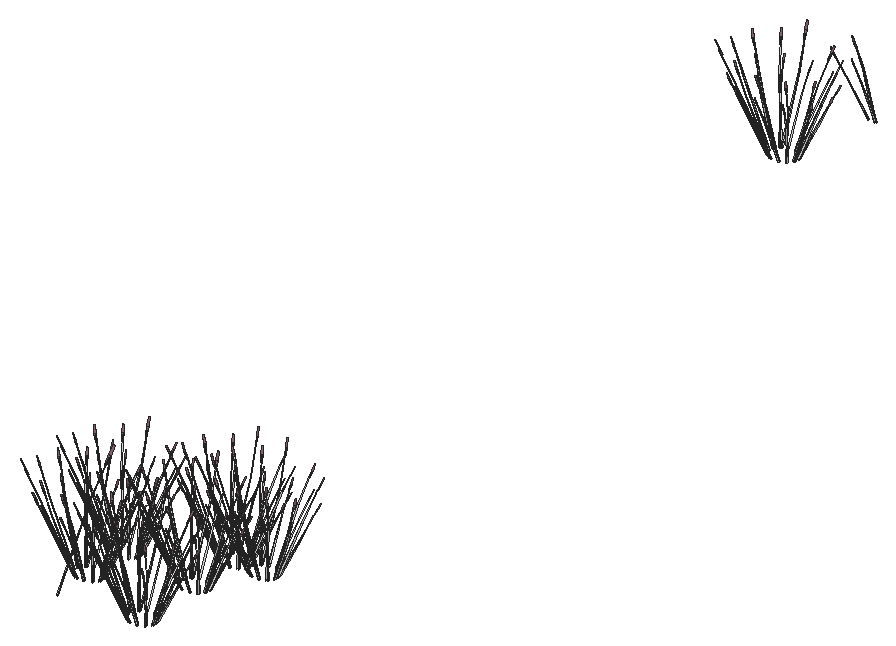
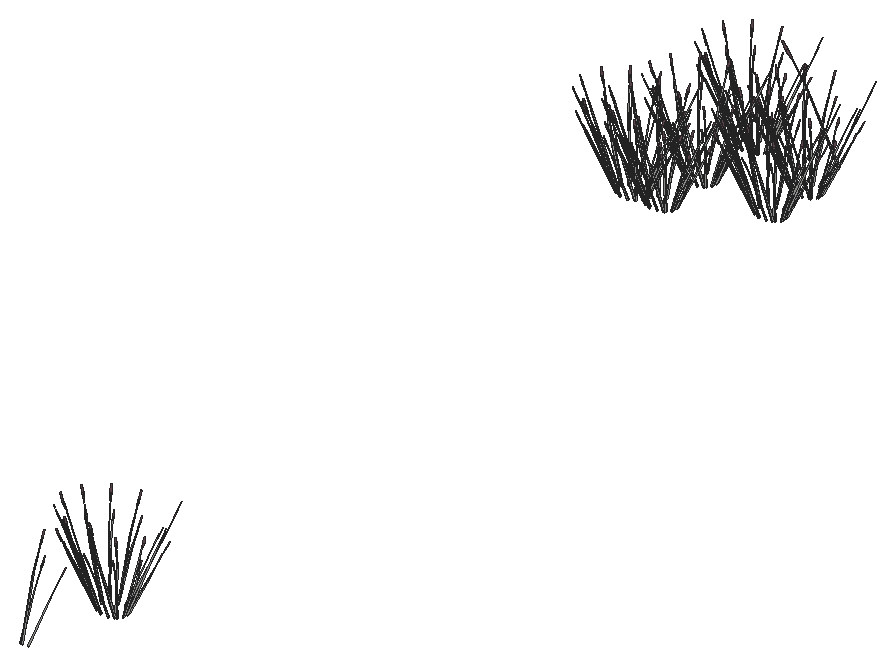
# SketchUp Ruby script. Lengths in inches.
U = 1.inch
M = Sketchup.active_model
def pt(a) = Geom::Point3d.new(a.map { |v| v * U })
def face(e, loops, mat)
  f = e.add_face(loops[0].map { |a| pt(a) })
  loops[1..].each { |l| e.add_face(l.map { |a| pt(a) }).erase! }
  f.material = f.back_material = mat if mat
  f
end
# faces: each face lists its corners as indices into pts; further lists are holes
def faces(e, pts, list, mat = nil) = list.each { |f| face(e, (f[0].is_a?(Array) ? f : [f]).map { |l| l.map { |i| pts[i] } }, mat) }
# xy, xz, yz: faces in a plane at the given z, y or x. An outline is a flat list of corners, or four numbers for a rectangle; further outlines are holes
def ring(l) = l.size == 4 ? [[l[0], l[1]], [l[2], l[1]], [l[2], l[3]], [l[0], l[3]]] : l.each_slice(2).to_a
def flat(e, list, mat, &to3) = list.each { |f| face(e, (f[0].is_a?(Array) ? f : [f]).map { |l| ring(l).map { |u, v| to3.(u, v) } }, mat) }
def xy(e, z, list, mat = nil) = flat(e, list, mat) { |x, y| [x, y, z] }
def xz(e, y, list, mat = nil) = flat(e, list, mat) { |x, z| [x, y, z] }
def yz(e, x, list, mat = nil) = flat(e, list, mat) { |y, z| [x, y, z] }
def lines(e, pts, list) = list.each { |a, b| e.add_line(pt(pts[a]), pt(pts[b])) }
# prism: a flat outline (further loops are holes) pulled along v
def prism(e, loops, v, mat = nil)
  f = face(e, loops, mat); d = Geom::Vector3d.new(v.map { |x| x * U })
  f.pushpull(f.normal.samedirection?(d) ? d.length : -d.length)
end
def box(e, o, s, mat = nil) = prism(e, [[o, [o[0] + s[0], o[1], o[2]], [o[0] + s[0], o[1] + s[1], o[2]], [o[0], o[1] + s[1], o[2]]]], [0, 0, s[2]], mat)
def at(x, y, z, deg = 0) = Geom::Transformation.translation(pt([x, y, z])) * Geom::Transformation.rotation(ORIGIN, Z_AXIS, deg.degrees)
def axes(o, x, y, z) = Geom::Transformation.new([*x, 0, *y, 0, *z, 0, *pt(o).to_a, 1])
def part(name) = M.definitions.add(name)
# library, detail: a bought-in or finely detailed component or shape, given as its bounding box
def library(name, o, s) = part(name).tap { |d| box(d.entities, o, s) }
def detail(e, o, s) = box(e.add_group.entities, o, s)
def put(e, d, t, mat = nil) = e.add_instance(d, t).tap { |i| i.material = mat if mat }
def group(e, t, mat = nil) = e.add_group.tap { |g| g.transformation = t; g.material = mat if mat }.entities
root = M.entities
M.materials.add("LightPink_Translucent").color = [144, 107, 117]
c1 = part("blade")
p = [[2.15,0.21,22],[0,0.17,0],[0.09,0.45,0],[2.18,0.31,22],[2.29,0.31,22],[0.38,0.45,0],
  [2.48,0.24,33],[2.49,0.24,33],[2.48,0.22,33]]
faces(c1.entities,p,[[0,1,2,3],[4,5,2,3],[6,3,4,7],[8,0,3,6]])
c2 = part("seeds")
p = [[0.3,-0.1,1.38],[-0.01,-0.03,1.59],[-0.01,-0.03,0.03],[0.14,-0.07,-0.07],[0.29,-0.03,3],[0.15,0.01,3.11]]
faces(c2.entities,p,[[0,1,2,3],[1,0,4,5]],"LightPink_Translucent")
c3 = part("blade with seeds")
put(c3.entities,c1,at(0,0,0))
put(c3.entities,c2,axes([2.4,0.25,30.99],[1.5799,-0.05474,1.17369],[-0.12525,1.92788,0.29478],[-0.07173,-0.02425,1.56792]))
put(root,c3,axes([64.49,21.74,46.73],[1.20755,0.27075,0.48003],[-0.41292,0.89013,0.3958],[-0.07257,-0.35005,0.9933]))
put(root,c3,axes([64.8125,21.67,46.73],[0.90301,-0.35198,0.0643],[0.44199,0.64184,0.50621],[-0.08721,-0.28293,0.77189]))
put(root,c3,axes([61.72,21.77,46.73],[0.55698,-0.6579,0.0643],[0.79316,0.38303,0.50621],[-0.25643,-0.21093,0.77189]))
put(root,c3,axes([67.23,22.73,46.73],[0.87265,0.70663,0.48003],[-0.92674,0.60943,0.3958],[0.16097,-0.33153,0.9933]))
put(root,c3,axes([61.97,21.7,47.43],[-0.81789,0.99285,-0.13619],[-1.18445,-0.572,-0.75594],[-0.41173,-0.28051,1.14864]))
put(root,c3,axes([67.55,22.8,46.73],[1.00708,0.04826,0.0643],[-0.02761,0.72867,0.50621],[0.10538,-0.27912,0.77189]))
put(root,c3,axes([59.1,23.0625,46.73],[0.06171,-0.78753,0.0643],[0.9318,0.02159,0.50621],[-0.35694,-0.08241,0.77189]))
put(root,c3,axes([69.21,24.84,46.73],[0.8413,0.43556,0.0643],[-0.48981,0.62025,0.50621],[0.26973,-0.20053,0.77189]))
put(root,c3,axes([68.97,24.66,46.73],[0.30393,0.95317,0.48003],[-1.19224,0.16542,0.3958],[0.35138,-0.22417,0.9933]))
put(root,c3,axes([57.75,25.46,46.73],[0.34623,-0.9443,0.48003],[1.13828,0.3229,0.3958],[-0.44763,0.05675,0.9933]))
put(root,c3,axes([57.66,25.21,46.73],[-0.4501,-0.70615,0.0643],[0.82077,-0.34564,0.50621],[-0.36181,0.0682,0.77189]))
put(root,c3,axes([69.33,27.26,46.73],[0.4501,0.70615,0.0643],[-0.82077,0.34564,0.50621],[0.36181,-0.0682,0.77189]))
put(root,c3,axes([69.25,27.01,46.73],[-0.34623,0.9443,0.48003],[-1.13828,-0.3229,0.3958],[0.44763,-0.05675,0.9933]))
put(root,c3,axes([33.02,33.74,46.73],[1.20755,0.27075,0.48003],[-0.41292,0.89013,0.3958],[-0.07257,-0.35005,0.9933]))
put(root,c3,axes([33.34,33.67,46.73],[0.90301,-0.35198,0.0643],[0.44199,0.64184,0.50621],[-0.08721,-0.28293,0.77189]))
put(root,c3,axes([30.25,33.77,46.73],[0.55698,-0.6579,0.0643],[0.79316,0.38303,0.50621],[-0.25643,-0.21093,0.77189]))
put(root,c3,axes([32.82,21.08,46.72],[-1.05895,-0.53811,1.38283],[1.11816,-0.83781,0.59665],[0.34166,0.5049,1.33663]))
put(root,c3,axes([35.76,34.73,46.73],[0.87265,0.70663,0.48003],[-0.92674,0.60943,0.3958],[0.16097,-0.33153,0.9933]))
put(root,c3,axes([30.5,33.7,47.43],[-0.81789,0.99285,-0.13619],[-1.18445,-0.572,-0.75594],[-0.41173,-0.28051,1.14864]))
put(root,c3,axes([36.08,34.8,46.73],[1.00708,0.04826,0.0643],[-0.02761,0.72867,0.50621],[0.10538,-0.27912,0.77189]))
put(root,c3,axes([58.02,27.81,46.73],[-0.30393,-0.95317,0.48003],[1.19224,-0.16542,0.3958],[-0.35138,0.22417,0.9933]))
put(root,c3,axes([57.79,27.63,46.73],[-0.8413,-0.43556,0.0643],[0.48981,-0.62025,0.50621],[-0.26973,0.20053,0.77189]))
put(root,c3,axes([67.9,29.4,46.73],[-0.06171,0.78753,0.0643],[-0.9318,-0.02159,0.50621],[0.35694,0.08241,0.77189]))
put(root,c3,axes([67.98,29.15,46.73],[-0.90362,0.68241,0.48003],[-0.77932,-0.72471,0.3958],[0.42395,0.12588,0.9933]))
put(root,c3,axes([27.63,35.0625,46.73],[0.06171,-0.78753,0.0643],[0.9318,0.02159,0.50621],[-0.35694,-0.08241,0.77189]))
put(root,c3,axes([37.74,36.84,46.73],[0.8413,0.43556,0.0643],[-0.48981,0.62025,0.50621],[0.26973,-0.20053,0.77189]))
put(root,c3,axes([37.5,36.66,46.73],[0.30393,0.95317,0.48003],[-1.19224,0.16542,0.3958],[0.35138,-0.22417,0.9933]))
put(root,c3,axes([59.44,29.67,46.73],[-1.00708,-0.04826,0.0643],[0.02761,-0.72867,0.50621],[-0.10538,0.27912,0.77189]))
put(root,c3,axes([59.77,29.74,46.73],[-0.87265,-0.70663,0.48003],[0.92674,-0.60943,0.3958],[-0.16097,0.33153,0.9933]))
put(root,c3,axes([65.28,30.7,46.73],[-0.55698,0.6579,0.0643],[-0.79316,-0.38303,0.50621],[0.25643,0.21093,0.77189]))
put(root,c3,axes([65.51,30.52,46.73],[-1.21888,0.23767,0.48003],[-0.21154,-0.93233,0.3958],[0.28666,0.27478,0.9933]))
put(root,c3,axes([62.1875,30.8,46.73],[-0.90301,0.35198,0.0643],[-0.44199,-0.64184,0.50621],[0.08721,0.28293,0.77189]))
put(root,c3,axes([59.67,29.33,47.4],[1.34686,0.05131,-0.13498],[-0.03681,0.97156,-0.74919],[-0.09356,0.37418,1.13838]))
put(root,c3,axes([26.28,37.46,46.73],[0.34623,-0.9443,0.48003],[1.13828,0.3229,0.3958],[-0.44763,0.05675,0.9933]))
put(root,c3,axes([26.19,37.21,46.73],[-0.4501,-0.70615,0.0643],[0.82077,-0.34564,0.50621],[-0.36181,0.0682,0.77189]))
put(root,c3,axes([37.86,39.26,46.73],[0.4501,0.70615,0.0643],[-0.82077,0.34564,0.50621],[0.36181,-0.0682,0.77189]))
put(root,c3,axes([37.78,39.01,46.73],[-0.34623,0.9443,0.48003],[-1.13828,-0.3229,0.3958],[0.44763,-0.05675,0.9933]))
put(root,c3,axes([26.55,39.81,46.73],[-0.30393,-0.95317,0.48003],[1.19224,-0.16542,0.3958],[-0.35138,0.22417,0.9933]))
put(root,c3,axes([26.32,39.63,46.73],[-0.8413,-0.43556,0.0643],[0.48981,-0.62025,0.50621],[-0.26973,0.20053,0.77189]))
put(root,c3,axes([64.28,49.02,46.73],[1.20755,0.27075,0.48003],[-0.41292,0.89013,0.3958],[-0.07257,-0.35005,0.9933]))
put(root,c3,axes([64.6,48.96,46.73],[0.90301,-0.35198,0.0643],[0.44199,0.64184,0.50621],[-0.08721,-0.28293,0.77189]))
put(root,c3,axes([36.42,41.4,46.73],[-0.06171,0.78753,0.0643],[-0.9318,-0.02159,0.50621],[0.35694,0.08241,0.77189]))
put(root,c3,axes([36.51,41.15,46.73],[-0.90362,0.68241,0.48003],[-0.77932,-0.72471,0.3958],[0.42395,0.12588,0.9933]))
put(root,c3,axes([61.51,49.06,46.73],[0.55698,-0.6579,0.0643],[0.79316,0.38303,0.50621],[-0.25643,-0.21093,0.77189]))
put(root,c3,axes([67.02,50.01,46.73],[0.87265,0.70663,0.48003],[-0.92674,0.60943,0.3958],[0.16097,-0.33153,0.9933]))
put(root,c3,axes([61.76,48.99,47.43],[-0.81789,0.99285,-0.13619],[-1.18445,-0.572,-0.75594],[-0.41173,-0.28051,1.14864]))
put(root,c3,axes([67.35,50.08,46.73],[1.00708,0.04826,0.0643],[-0.02761,0.72867,0.50621],[0.10538,-0.27912,0.77189]))
put(root,c3,axes([27.97,41.67,46.73],[-1.00708,-0.04826,0.0643],[0.02761,-0.72867,0.50621],[-0.10538,0.27912,0.77189]))
put(root,c3,axes([28.29,41.74,46.73],[-0.87265,-0.70663,0.48003],[0.92674,-0.60943,0.3958],[-0.16097,0.33153,0.9933]))
put(root,c3,axes([32.72,52.77,46.73],[1.20755,0.27075,0.48003],[-0.41292,0.89013,0.3958],[-0.07257,-0.35005,0.9933]))
put(root,c3,axes([33.04,52.7,46.73],[0.90301,-0.35198,0.0643],[0.44199,0.64184,0.50621],[-0.08721,-0.28293,0.77189]))
put(root,c3,axes([33.81,42.7,46.73],[-0.55698,0.6579,0.0643],[-0.79316,-0.38303,0.50621],[0.25643,0.21093,0.77189]))
put(root,c3,axes([34.04,42.52,46.73],[-1.21888,0.23767,0.48003],[-0.21154,-0.93233,0.3958],[0.28666,0.27478,0.9933]))
put(root,c3,axes([58.89,50.35,46.73],[0.06171,-0.78753,0.0643],[0.9318,0.02159,0.50621],[-0.35694,-0.08241,0.77189]))
put(root,c3,axes([29.95,52.8,46.73],[0.55698,-0.6579,0.0643],[0.79316,0.38303,0.50621],[-0.25643,-0.21093,0.77189]))
put(root,c3,axes([30.71,42.8,46.73],[-0.90301,0.35198,0.0643],[-0.44199,-0.64184,0.50621],[0.08721,0.28293,0.77189]))
put(root,c3,axes([28.2,41.33,47.4],[1.34686,0.05131,-0.13498],[-0.03681,0.97156,-0.74919],[-0.09356,0.37418,1.13838]))
put(root,c3,axes([35.46,53.76,46.73],[0.87265,0.70663,0.48003],[-0.92674,0.60943,0.3958],[0.16097,-0.33153,0.9933]))
put(root,c3,axes([30.2,52.73,47.43],[-0.81789,0.99285,-0.13619],[-1.18445,-0.572,-0.75594],[-0.41173,-0.28051,1.14864]))
put(root,c3,axes([35.78,53.82,46.73],[1.00708,0.04826,0.0643],[-0.02761,0.72867,0.50621],[0.10538,-0.27912,0.77189]))
put(root,c3,axes([69,52.13,46.73],[0.8413,0.43556,0.0643],[-0.48981,0.62025,0.50621],[0.26973,-0.20053,0.77189]))
put(root,c3,axes([68.77,51.94,46.73],[0.30393,0.95317,0.48003],[-1.19224,0.16542,0.3958],[0.35138,-0.22417,0.9933]))
put(root,c3,axes([27.33,54.09,46.73],[0.06171,-0.78753,0.0643],[0.9318,0.02159,0.50621],[-0.35694,-0.08241,0.77189]))
put(root,c3,axes([57.54,52.74,46.73],[0.34623,-0.9443,0.48003],[1.13828,0.3229,0.3958],[-0.44763,0.05675,0.9933]))
put(root,c3,axes([57.46,52.49,46.73],[-0.4501,-0.70615,0.0643],[0.82077,-0.34564,0.50621],[-0.36181,0.0682,0.77189]))
put(root,c3,axes([37.4375,55.87,46.73],[0.8413,0.43556,0.0643],[-0.48981,0.62025,0.50621],[0.26973,-0.20053,0.77189]))
put(root,c3,axes([37.2,55.6875,46.73],[0.30393,0.95317,0.48003],[-1.19224,0.16542,0.3958],[0.35138,-0.22417,0.9933]))
put(root,c3,axes([69.125,54.55,46.73],[0.4501,0.70615,0.0643],[-0.82077,0.34564,0.50621],[0.36181,-0.0682,0.77189]))
put(root,c3,axes([69.04,54.3,46.73],[-0.34623,0.9443,0.48003],[-1.13828,-0.3229,0.3958],[0.44763,-0.05675,0.9933]))
put(root,c3,axes([25.98,56.49,46.73],[0.34623,-0.9443,0.48003],[1.13828,0.3229,0.3958],[-0.44763,0.05675,0.9933]))
put(root,c3,axes([25.89,56.24,46.73],[-0.4501,-0.70615,0.0643],[0.82077,-0.34564,0.50621],[-0.36181,0.0682,0.77189]))
put(root,c3,axes([57.82,55.1,46.73],[-0.30393,-0.95317,0.48003],[1.19224,-0.16542,0.3958],[-0.35138,0.22417,0.9933]))
put(root,c3,axes([57.58,54.91,46.73],[-0.8413,-0.43556,0.0643],[0.48981,-0.62025,0.50621],[-0.26973,0.20053,0.77189]))
put(root,c3,axes([37.5625,58.29,46.73],[0.4501,0.70615,0.0643],[-0.82077,0.34564,0.50621],[0.36181,-0.0682,0.77189]))
put(root,c3,axes([37.48,58.04,46.73],[-0.34623,0.9443,0.48003],[-1.13828,-0.3229,0.3958],[0.44763,-0.05675,0.9933]))
put(root,c3,axes([67.6875,56.69,46.73],[-0.06171,0.78753,0.0643],[-0.9318,-0.02159,0.50621],[0.35694,0.08241,0.77189]))
put(root,c3,axes([67.77,56.44,46.73],[-0.90362,0.68241,0.48003],[-0.77932,-0.72471,0.3958],[0.42395,0.12588,0.9933]))
put(root,c3,axes([26.25,58.84,46.73],[-0.30393,-0.95317,0.48003],[1.19224,-0.16542,0.3958],[-0.35138,0.22417,0.9933]))
put(root,c3,axes([26.02,58.66,46.73],[-0.8413,-0.43556,0.0643],[0.48981,-0.62025,0.50621],[-0.26973,0.20053,0.77189]))
put(root,c3,axes([59.24,56.96,46.73],[-1.00708,-0.04826,0.0643],[0.02761,-0.72867,0.50621],[-0.10538,0.27912,0.77189]))
put(root,c3,axes([59.56,57.03,46.73],[-0.87265,-0.70663,0.48003],[0.92674,-0.60943,0.3958],[-0.16097,0.33153,0.9933]))
put(root,c3,axes([65.07,57.99,46.73],[-0.55698,0.6579,0.0643],[-0.79316,-0.38303,0.50621],[0.25643,0.21093,0.77189]))
put(root,c3,axes([65.31,57.8,46.73],[-1.21888,0.23767,0.48003],[-0.21154,-0.93233,0.3958],[0.28666,0.27478,0.9933]))
put(root,c3,axes([36.125,60.43,46.73],[-0.06171,0.78753,0.0643],[-0.9318,-0.02159,0.50621],[0.35694,0.08241,0.77189]))
put(root,c3,axes([36.21,60.18,46.73],[-0.90362,0.68241,0.48003],[-0.77932,-0.72471,0.3958],[0.42395,0.12588,0.9933]))
put(root,c3,axes([61.98,58.08,46.73],[-0.90301,0.35198,0.0643],[-0.44199,-0.64184,0.50621],[0.08721,0.28293,0.77189]))
put(root,c3,axes([59.46,56.61,47.4],[1.34686,0.05131,-0.13498],[-0.03681,0.97156,-0.74919],[-0.09356,0.37418,1.13838]))
put(root,c3,axes([64.28,69.74,46.73],[1.20755,0.27075,0.48003],[-0.41292,0.89013,0.3958],[-0.07257,-0.35005,0.9933]))
put(root,c3,axes([76.28,69.74,46.73],[1.20755,0.27075,0.48003],[-0.41292,0.89013,0.3958],[-0.07257,-0.35005,0.9933]))
put(root,c3,axes([64.6,69.67,46.73],[0.90301,-0.35198,0.0643],[0.44199,0.64184,0.50621],[-0.08721,-0.28293,0.77189]))
put(root,c3,axes([76.6,69.67,46.73],[0.90301,-0.35198,0.0643],[0.44199,0.64184,0.50621],[-0.08721,-0.28293,0.77189]))
put(root,c3,axes([61.51,69.77,46.73],[0.55698,-0.6579,0.0643],[0.79316,0.38303,0.50621],[-0.25643,-0.21093,0.77189]))
put(root,c3,axes([73.51,69.77,46.73],[0.55698,-0.6579,0.0643],[0.79316,0.38303,0.50621],[-0.25643,-0.21093,0.77189]))
put(root,c3,axes([27.67,60.7,46.73],[-1.00708,-0.04826,0.0643],[0.02761,-0.72867,0.50621],[-0.10538,0.27912,0.77189]))
put(root,c3,axes([28,60.77,46.73],[-0.87265,-0.70663,0.48003],[0.92674,-0.60943,0.3958],[-0.16097,0.33153,0.9933]))
put(root,c3,axes([67.02,70.73,46.73],[0.87265,0.70663,0.48003],[-0.92674,0.60943,0.3958],[0.16097,-0.33153,0.9933]))
put(root,c3,axes([79.02,70.73,46.73],[0.87265,0.70663,0.48003],[-0.92674,0.60943,0.3958],[0.16097,-0.33153,0.9933]))
put(root,c3,axes([61.76,69.7,47.43],[-0.81789,0.99285,-0.13619],[-1.18445,-0.572,-0.75594],[-0.41173,-0.28051,1.14864]))
put(root,c3,axes([73.76,69.7,47.43],[-0.81789,0.99285,-0.13619],[-1.18445,-0.572,-0.75594],[-0.41173,-0.28051,1.14864]))
put(root,c3,axes([67.35,70.8,46.73],[1.00708,0.04826,0.0643],[-0.02761,0.72867,0.50621],[0.10538,-0.27912,0.77189]))
put(root,c3,axes([79.35,70.8,46.73],[1.00708,0.04826,0.0643],[-0.02761,0.72867,0.50621],[0.10538,-0.27912,0.77189]))
put(root,c3,axes([33.51,61.73,46.73],[-0.55698,0.6579,0.0643],[-0.79316,-0.38303,0.50621],[0.25643,0.21093,0.77189]))
put(root,c3,axes([33.74,61.55,46.73],[-1.21888,0.23767,0.48003],[-0.21154,-0.93233,0.3958],[0.28666,0.27478,0.9933]))
put(root,c3,axes([30.42,61.83,46.73],[-0.90301,0.35198,0.0643],[-0.44199,-0.64184,0.50621],[0.08721,0.28293,0.77189]))
put(root,c3,axes([27.9,60.36,47.4],[1.34686,0.05131,-0.13498],[-0.03681,0.97156,-0.74919],[-0.09356,0.37418,1.13838]))
put(root,c3,axes([58.89,71.0625,46.73],[0.06171,-0.78753,0.0643],[0.9318,0.02159,0.50621],[-0.35694,-0.08241,0.77189]))
put(root,c3,axes([70.89,71.0625,46.73],[0.06171,-0.78753,0.0643],[0.9318,0.02159,0.50621],[-0.35694,-0.08241,0.77189]))
put(root,c3,axes([69,72.84,46.73],[0.8413,0.43556,0.0643],[-0.48981,0.62025,0.50621],[0.26973,-0.20053,0.77189]))
put(root,c3,axes([81,72.84,46.73],[0.8413,0.43556,0.0643],[-0.48981,0.62025,0.50621],[0.26973,-0.20053,0.77189]))
put(root,c3,axes([68.77,72.66,46.73],[0.30393,0.95317,0.48003],[-1.19224,0.16542,0.3958],[0.35138,-0.22417,0.9933]))
put(root,c3,axes([80.77,72.66,46.73],[0.30393,0.95317,0.48003],[-1.19224,0.16542,0.3958],[0.35138,-0.22417,0.9933]))
put(root,c3,axes([57.54,73.46,46.73],[0.34623,-0.9443,0.48003],[1.13828,0.3229,0.3958],[-0.44763,0.05675,0.9933]))
put(root,c3,axes([69.54,73.46,46.73],[0.34623,-0.9443,0.48003],[1.13828,0.3229,0.3958],[-0.44763,0.05675,0.9933]))
put(root,c3,axes([57.46,73.21,46.73],[-0.4501,-0.70615,0.0643],[0.82077,-0.34564,0.50621],[-0.36181,0.0682,0.77189]))
put(root,c3,axes([69.46,73.21,46.73],[-0.4501,-0.70615,0.0643],[0.82077,-0.34564,0.50621],[-0.36181,0.0682,0.77189]))
put(root,c3,axes([69.125,75.26,46.73],[0.4501,0.70615,0.0643],[-0.82077,0.34564,0.50621],[0.36181,-0.0682,0.77189]))
put(root,c3,axes([81.125,75.26,46.73],[0.4501,0.70615,0.0643],[-0.82077,0.34564,0.50621],[0.36181,-0.0682,0.77189]))
put(root,c3,axes([69.04,75.01,46.73],[-0.34623,0.9443,0.48003],[-1.13828,-0.3229,0.3958],[0.44763,-0.05675,0.9933]))
put(root,c3,axes([81.04,75.01,46.73],[-0.34623,0.9443,0.48003],[-1.13828,-0.3229,0.3958],[0.44763,-0.05675,0.9933]))
put(root,c3,axes([57.82,75.81,46.73],[-0.30393,-0.95317,0.48003],[1.19224,-0.16542,0.3958],[-0.35138,0.22417,0.9933]))
put(root,c3,axes([69.82,75.81,46.73],[-0.30393,-0.95317,0.48003],[1.19224,-0.16542,0.3958],[-0.35138,0.22417,0.9933]))
put(root,c3,axes([57.58,75.63,46.73],[-0.8413,-0.43556,0.0643],[0.48981,-0.62025,0.50621],[-0.26973,0.20053,0.77189]))
put(root,c3,axes([69.58,75.63,46.73],[-0.8413,-0.43556,0.0643],[0.48981,-0.62025,0.50621],[-0.26973,0.20053,0.77189]))
put(root,c3,axes([67.6875,77.4,46.73],[-0.06171,0.78753,0.0643],[-0.9318,-0.02159,0.50621],[0.35694,0.08241,0.77189]))
put(root,c3,axes([79.6875,77.4,46.73],[-0.06171,0.78753,0.0643],[-0.9318,-0.02159,0.50621],[0.35694,0.08241,0.77189]))
put(root,c3,axes([67.77,77.15,46.73],[-0.90362,0.68241,0.48003],[-0.77932,-0.72471,0.3958],[0.42395,0.12588,0.9933]))
put(root,c3,axes([79.77,77.15,46.73],[-0.90362,0.68241,0.48003],[-0.77932,-0.72471,0.3958],[0.42395,0.12588,0.9933]))
put(root,c3,axes([59.24,77.67,46.73],[-1.00708,-0.04826,0.0643],[0.02761,-0.72867,0.50621],[-0.10538,0.27912,0.77189]))
put(root,c3,axes([71.24,77.67,46.73],[-1.00708,-0.04826,0.0643],[0.02761,-0.72867,0.50621],[-0.10538,0.27912,0.77189]))
put(root,c3,axes([59.56,77.74,46.73],[-0.87265,-0.70663,0.48003],[0.92674,-0.60943,0.3958],[-0.16097,0.33153,0.9933]))
put(root,c3,axes([71.56,77.74,46.73],[-0.87265,-0.70663,0.48003],[0.92674,-0.60943,0.3958],[-0.16097,0.33153,0.9933]))
put(root,c3,axes([65.07,78.7,46.73],[-0.55698,0.6579,0.0643],[-0.79316,-0.38303,0.50621],[0.25643,0.21093,0.77189]))
put(root,c3,axes([77.07,78.7,46.73],[-0.55698,0.6579,0.0643],[-0.79316,-0.38303,0.50621],[0.25643,0.21093,0.77189]))
put(root,c3,axes([65.31,78.52,46.73],[-1.21888,0.23767,0.48003],[-0.21154,-0.93233,0.3958],[0.28666,0.27478,0.9933]))
put(root,c3,axes([77.31,78.52,46.73],[-1.21888,0.23767,0.48003],[-0.21154,-0.93233,0.3958],[0.28666,0.27478,0.9933]))
put(root,c3,axes([61.98,78.8,46.73],[-0.90301,0.35198,0.0643],[-0.44199,-0.64184,0.50621],[0.08721,0.28293,0.77189]))
put(root,c3,axes([73.98,78.8,46.73],[-0.90301,0.35198,0.0643],[-0.44199,-0.64184,0.50621],[0.08721,0.28293,0.77189]))
put(root,c3,axes([59.46,77.33,47.4],[1.34686,0.05131,-0.13498],[-0.03681,0.97156,-0.74919],[-0.09356,0.37418,1.13838]))
put(root,c3,axes([71.46,77.33,47.4],[1.34686,0.05131,-0.13498],[-0.03681,0.97156,-0.74919],[-0.09356,0.37418,1.13838]))
put(root,c3,axes([35.44,388.48,46.73],[1.20755,0.27075,0.48003],[-0.41292,0.89013,0.3958],[-0.07257,-0.35005,0.9933]))
put(root,c3,axes([35.76,388.41,46.73],[0.90301,-0.35198,0.0643],[0.44199,0.64184,0.50621],[-0.08721,-0.28293,0.77189]))
put(root,c3,axes([32.67,388.51,46.73],[0.55698,-0.6579,0.0643],[0.79316,0.38303,0.50621],[-0.25643,-0.21093,0.77189]))
put(root,c3,axes([38.18,389.47,46.73],[0.87265,0.70663,0.48003],[-0.92674,0.60943,0.3958],[0.16097,-0.33153,0.9933]))
put(root,c3,axes([32.92,388.4375,47.43],[-0.81789,0.99285,-0.13619],[-1.18445,-0.572,-0.75594],[-0.41173,-0.28051,1.14864]))
put(root,c3,axes([38.5,389.53,46.73],[1.00708,0.04826,0.0643],[-0.02761,0.72867,0.50621],[0.10538,-0.27912,0.77189]))
put(root,c3,axes([30.05,389.8,46.73],[0.06171,-0.78753,0.0643],[0.9318,0.02159,0.50621],[-0.35694,-0.08241,0.77189]))
put(root,c3,axes([40.16,391.58,46.73],[0.8413,0.43556,0.0643],[-0.48981,0.62025,0.50621],[0.26973,-0.20053,0.77189]))
put(root,c3,axes([39.93,391.4,46.73],[0.30393,0.95317,0.48003],[-1.19224,0.16542,0.3958],[0.35138,-0.22417,0.9933]))
put(root,c3,axes([28.7,392.2,46.73],[0.34623,-0.9443,0.48003],[1.13828,0.3229,0.3958],[-0.44763,0.05675,0.9933]))
put(root,c3,axes([28.61,391.95,46.73],[-0.4501,-0.70615,0.0643],[0.82077,-0.34564,0.50621],[-0.36181,0.0682,0.77189]))
put(root,c3,axes([40.29,394,46.73],[0.4501,0.70615,0.0643],[-0.82077,0.34564,0.50621],[0.36181,-0.0682,0.77189]))
put(root,c3,axes([40.2,393.75,46.73],[-0.34623,0.9443,0.48003],[-1.13828,-0.3229,0.3958],[0.44763,-0.05675,0.9933]))
put(root,c3,axes([28.98,394.55,46.73],[-0.30393,-0.95317,0.48003],[1.19224,-0.16542,0.3958],[-0.35138,0.22417,0.9933]))
put(root,c3,axes([28.74,394.37,46.73],[-0.8413,-0.43556,0.0643],[0.48981,-0.62025,0.50621],[-0.26973,0.20053,0.77189]))
put(root,c3,axes([38.85,396.14,46.73],[-0.06171,0.78753,0.0643],[-0.9318,-0.02159,0.50621],[0.35694,0.08241,0.77189]))
put(root,c3,axes([38.93,395.89,46.73],[-0.90362,0.68241,0.48003],[-0.77932,-0.72471,0.3958],[0.42395,0.12588,0.9933]))
put(root,c3,axes([30.4,396.41,46.73],[-1.00708,-0.04826,0.0643],[0.02761,-0.72867,0.50621],[-0.10538,0.27912,0.77189]))
put(root,c3,axes([30.72,396.48,46.73],[-0.87265,-0.70663,0.48003],[0.92674,-0.60943,0.3958],[-0.16097,0.33153,0.9933]))
put(root,c3,axes([36.23,397.4375,46.73],[-0.55698,0.6579,0.0643],[-0.79316,-0.38303,0.50621],[0.25643,0.21093,0.77189]))
put(root,c3,axes([36.47,397.25,46.73],[-1.21888,0.23767,0.48003],[-0.21154,-0.93233,0.3958],[0.28666,0.27478,0.9933]))
put(root,c3,axes([33.14,397.54,46.73],[-0.90301,0.35198,0.0643],[-0.44199,-0.64184,0.50621],[0.08721,0.28293,0.77189]))
put(root,c3,axes([30.62,396.07,47.4],[1.34686,0.05131,-0.13498],[-0.03681,0.97156,-0.74919],[-0.09356,0.37418,1.13838]))
put(root,c3,axes([43.6,428.17,46.73],[1.20755,0.27075,0.48003],[-0.41292,0.89013,0.3958],[-0.07257,-0.35005,0.9933]))
put(root,c3,axes([43.92,428.1,46.73],[0.90301,-0.35198,0.0643],[0.44199,0.64184,0.50621],[-0.08721,-0.28293,0.77189]))
put(root,c3,axes([40.82,428.2,46.73],[0.55698,-0.6579,0.0643],[0.79316,0.38303,0.50621],[-0.25643,-0.21093,0.77189]))
